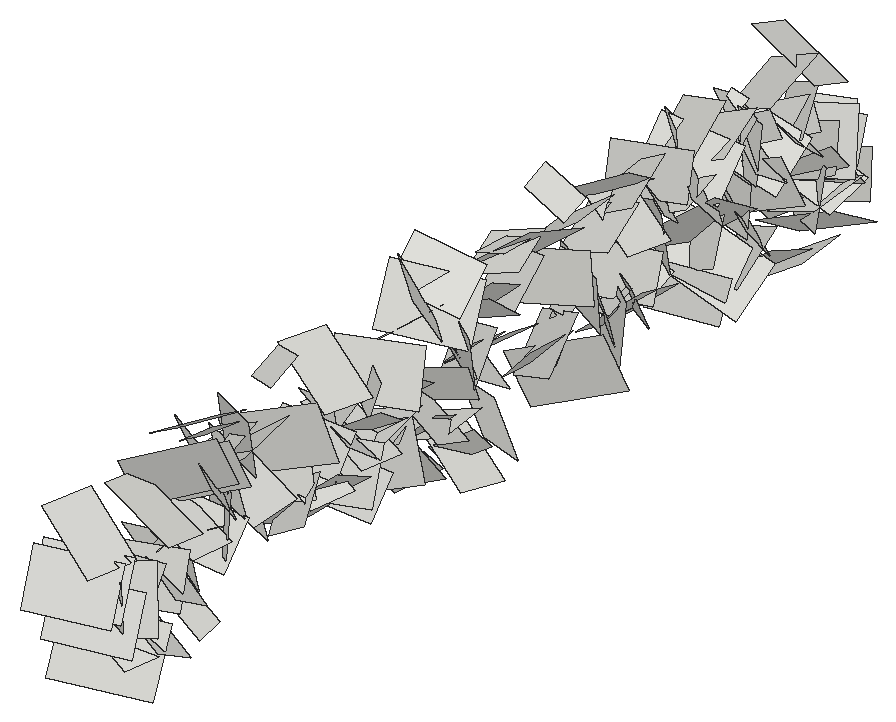
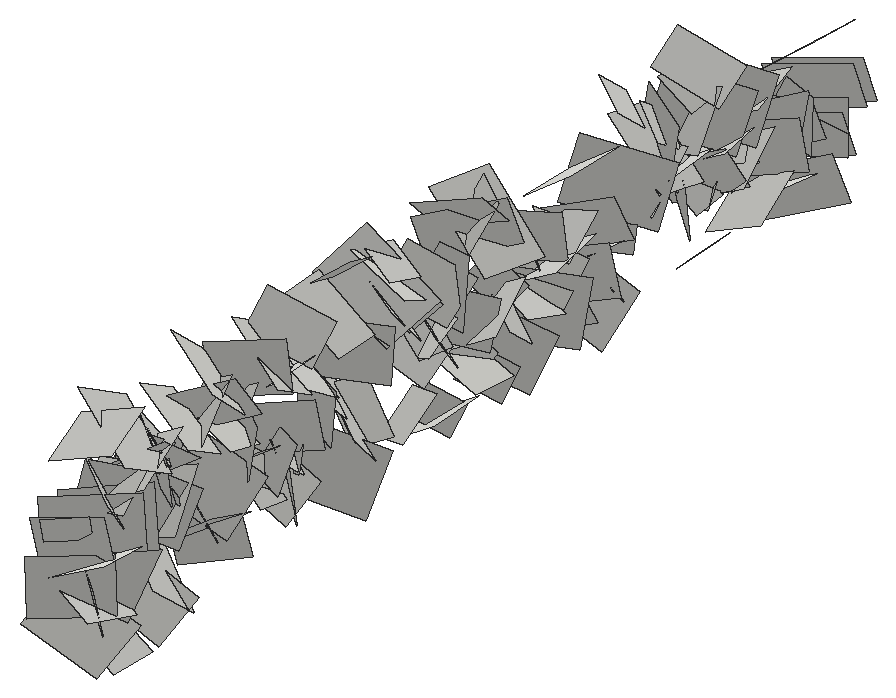
# SketchUp Ruby script. Lengths in inches.
U = 1.inch
M = Sketchup.active_model
def pt(a) = Geom::Point3d.new(a.map { |v| v * U })
def face(e, loops, mat)
  f = e.add_face(loops[0].map { |a| pt(a) })
  loops[1..].each { |l| e.add_face(l.map { |a| pt(a) }).erase! }
  f.material = f.back_material = mat if mat
  f
end
# faces: each face lists its corners as indices into pts; further lists are holes
def faces(e, pts, list, mat = nil) = list.each { |f| face(e, (f[0].is_a?(Array) ? f : [f]).map { |l| l.map { |i| pts[i] } }, mat) }
# xy, xz, yz: faces in a plane at the given z, y or x. An outline is a flat list of corners, or four numbers for a rectangle; further outlines are holes
def ring(l) = l.size == 4 ? [[l[0], l[1]], [l[2], l[1]], [l[2], l[3]], [l[0], l[3]]] : l.each_slice(2).to_a
def flat(e, list, mat, &to3) = list.each { |f| face(e, (f[0].is_a?(Array) ? f : [f]).map { |l| ring(l).map { |u, v| to3.(u, v) } }, mat) }
def xy(e, z, list, mat = nil) = flat(e, list, mat) { |x, y| [x, y, z] }
def xz(e, y, list, mat = nil) = flat(e, list, mat) { |x, z| [x, y, z] }
def yz(e, x, list, mat = nil) = flat(e, list, mat) { |y, z| [x, y, z] }
def lines(e, pts, list) = list.each { |a, b| e.add_line(pt(pts[a]), pt(pts[b])) }
# prism: a flat outline (further loops are holes) pulled along v
def prism(e, loops, v, mat = nil)
  f = face(e, loops, mat); d = Geom::Vector3d.new(v.map { |x| x * U })
  f.pushpull(f.normal.samedirection?(d) ? d.length : -d.length)
end
def box(e, o, s, mat = nil) = prism(e, [[o, [o[0] + s[0], o[1], o[2]], [o[0] + s[0], o[1] + s[1], o[2]], [o[0], o[1] + s[1], o[2]]]], [0, 0, s[2]], mat)
def at(x, y, z, deg = 0) = Geom::Transformation.translation(pt([x, y, z])) * Geom::Transformation.rotation(ORIGIN, Z_AXIS, deg.degrees)
def axes(o, x, y, z) = Geom::Transformation.new([*x, 0, *y, 0, *z, 0, *pt(o).to_a, 1])
def part(name) = M.definitions.add(name)
# library, detail: a bought-in or finely detailed component or shape, given as its bounding box
def library(name, o, s) = part(name).tap { |d| box(d.entities, o, s) }
def detail(e, o, s) = box(e.add_group.entities, o, s)
def put(e, d, t, mat = nil) = e.add_instance(d, t).tap { |i| i.material = mat if mat }
def group(e, t, mat = nil) = e.add_group.tap { |g| g.transformation = t; g.material = mat if mat }.entities
root = M.entities
c1 = part("Component\#6")
p = [[0.01,0,0],[0,3.24,4.54],[4.32,3.24,4.54],[4.33,0,0]]
faces(c1.entities,p,[[0,1,2,3]])
put(root,c1,axes([404.88,137.29,38.52],[0.00887,0.62519,-1.13199],[0.07674,-1.13046,-0.62381],[-1.3686,-0.05933,-0.04231]))
put(root,c1,axes([404.88,143.42,27.33],[-0.08667,-0.86973,1.01008],[0.23887,0.9884,0.86929],[-1.39256,0.22367,0.08625]))
put(root,c1,axes([404.88,132.16,25.41],[0.07094,-0.60211,-1.2376],[0.1162,-1.23279,0.6057],[-1.45423,-0.12788,-0.01197]))
put(root,c1,axes([404.88,172.47,36.95],[-0.1233,0.89549,0.4145],[-0.21728,0.38634,-0.89217],[-1.02316,-0.18996,0.13951]))
put(root,c1,axes([404.88,163.85,26.9],[-0.03329,1.04875,0.11229],[-0.24045,0.10299,-1.02538],[-1.09187,-0.05466,0.22238]))
put(root,c1,axes([404.88,195.34,33.06],[-0.01901,1.14103,-0.72029],[0.19621,-0.71146,-1.13165],[-1.41679,-0.11384,-0.14706]))
put(root,c1,axes([404.88,185.59,36.56],[-0.07365,1.00309,0.56692],[-0.00038,0.56794,-1.00493],[-1.22135,-0.06067,-0.03387]))
put(root,c1,axes([404.88,208.94,26.04],[0.1299,1.02121,-0.60997],[-0.25035,-0.5801,-1.01865],[-1.23578,0.22487,0.14225]))
put(root,c1,axes([404.88,141.2,30.22],[-0.14348,-0.5033,-0.91823],[-0.06175,-0.92081,0.51331],[-1.10823,0.11647,0.09028]))
put(root,c1,axes([404.88,196.35,35.86],[-0.06555,0.97369,0.5362],[-0.0688,0.53295,-0.97527],[-1.17625,-0.08544,0.02716]))
put(root,c1,axes([404.88,141.99,33.2],[-0.15631,-0.03731,1.01998],[-0.08418,1.02787,0.02612],[-1.07863,-0.07482,-0.14985]))
put(root,c1,axes([404.88,190.1,29],[-0.15352,-0.05709,1.12322],[0.06907,1.13017,0.06585],[-1.19015,0.07295,-0.14107]))
put(root,c1,axes([404.88,182.88,33.98],[-0.05541,0.90127,0.55592],[-0.17138,0.54328,-0.89597],[-1.1093,-0.12895,0.11065]))
put(root,c1,axes([404.88,146.73,29.36],[0.09029,-1.26195,0.03468],[-0.03892,0.03227,1.26436],[-1.33761,-0.08612,-0.03444]))
put(root,c1,axes([404.88,175.96,26.52],[-0.03553,0.82214,0.9074],[0.07429,0.90754,-0.81968],[-1.2958,0.02948,-0.07187]))
put(root,c1,axes([404.88,209.74,33.23],[-0.15201,0.07034,-1.21602],[0.20156,-1.20811,-0.09231],[-1.2753,-0.19933,0.13035]))
put(root,c1,axes([404.88,129.14,29.25],[0.07983,-0.47542,-1.06148],[-0.1788,-1.05692,0.46141],[-1.21984,0.1238,-0.1371]))
put(root,c1,axes([404.88,127.85,32.74],[0.07983,-0.47542,-1.06148],[-0.1788,-1.05692,0.46141],[-1.21984,0.1238,-0.1371]))
put(root,c1,axes([404.88,126.73,32.74],[0.07983,-0.47542,-1.06148],[-0.1788,-1.05692,0.46141],[-1.21984,0.1238,-0.1371]))
put(root,c1,axes([404.88,156.79,29.67],[-0.01777,-0.29003,-1.18393],[0.05362,-1.18318,0.28913],[-1.29096,-0.04516,0.0283]))
put(root,c1,axes([404.88,155.57,33.875],[-0.13701,-1.11756,0.11199],[0.07264,0.10468,1.12363],[-1.18833,0.13525,0.05577]))
put(root,c1,axes([404.88,151.45,29.33],[-0.11063,1.17252,-0.59491],[0.28501,-0.56514,-1.16101],[-1.36425,-0.21315,-0.19431]))
put(root,c1,axes([404.88,134.27,30.6],[-0.0256,-0.22889,-1.14247],[-0.00761,-1.14266,0.22909],[-1.23506,0.01178,0.02227]))
put(root,c1,axes([404.88,182.25,27.43],[0.1955,0.46825,-1.21407],[-0.10064,-1.21809,-0.48422],[-1.37564,0.15566,-0.13711]))
put(root,c1,axes([404.88,204.59,30.02],[0.04301,-1.09683,0.72238],[0.12053,0.72294,1.0913],[-1.38692,0.02882,0.11724]))
put(root,c1,axes([404.88,149.09,36.34],[0.1737,0.35213,-1.24285],[-0.08,-1.24806,-0.36356],[-1.36694,0.11779,-0.13666]))
put(root,c1,axes([404.88,180.75,35.09],[0.01445,0.08276,-1.11066],[-0.1396,-1.10283,-0.0838],[-1.17228,0.13235,-0.00371]))
put(root,c1,axes([404.88,201.85,37.73],[0.10519,1.13817,0.58904],[0.00109,0.59073,-1.14161],[-1.35845,0.08861,0.0447]))
put(root,c1,axes([404.88,198.78,35.93],[-0.06513,-0.64723,-0.92238],[-0.00055,-0.92374,0.64822],[-1.19442,0.03572,0.05]))
put(root,c1,axes([404.88,181.98,27.65],[-0.03848,-0.07343,1.06513],[-0.13392,1.05855,0.06867],[-1.12376,-0.12364,-0.04466]))
put(root,c1,axes([404.88,200.11,31.93],[-0.08158,0.26048,1.04137],[-0.05734,1.04178,-0.26458],[-1.13642,-0.07126,-0.06141]))
put(root,c1,axes([400.91,188.74,27.6],[-0.13014,-0.45431,-0.37588],[-0.00674,-0.3829,0.46487],[0.62498,-0.09873,-0.07326]))
put(root,c1,axes([404.88,153.58,31.99],[-0.17505,-0.32324,-0.90395],[-0.10086,-0.9072,0.34179],[-1.0126,0.14624,0.12223]))
put(root,c1,axes([400.91,136.62,23.89],[-0.08859,0.63974,0.04756],[-0.12242,0.03217,-0.63572],[0.66888,0.09062,-0.11005]))
put(root,c1,axes([404.88,213.06,27.02],[0.109,-1.16412,-0.17966],[-0.1638,-0.19212,1.15639],[-1.23778,-0.07709,-0.16885]))
put(root,c1,axes([404.88,137.65,40.3125],[-0.15365,0.92766,-0.3555],[-0.07441,-0.36793,-0.93147],[-1.05042,-0.10963,0.11798]))
put(root,c1,axes([404.88,201.95,25.76],[-0.02109,1.10253,-0.4508],[0.04504,-0.44992,-1.10225],[-1.2618,-0.03449,-0.03181]))
put(root,c1,axes([404.88,140.69,35.43],[-0.02714,1.22478,0.26938],[0.1382,0.27058,-1.21783],[-1.3221,0.00314,-0.13283]))
put(root,c1,axes([404.88,128.2,32.33],[-0.15852,-1.12421,0.05612],[0.12401,0.04078,1.12872],[-1.18668,0.15444,0.11046]))
put(root,c1,axes([404.88,138.43,27.8],[-0.10648,0.28124,1.16655],[0.16097,1.1642,-0.2676],[-1.26174,0.12479,-0.13259]))
put(root,c1,axes([404.88,157.84,26.69],[-0.16666,-0.37984,-0.88441],[-0.10341,-0.88523,0.39754],[-1.01503,0.15255,0.10471]))
put(root,c1,axes([404.88,213.59,29.33],[-0.10669,0.07311,-1.12569],[0.06812,-1.12796,-0.079],[-1.19381,-0.0709,0.09609]))
put(root,c1,axes([404.88,160.05,30.35],[0.12426,0.20575,-1.35522],[0.11745,-1.35714,-0.19646],[-1.44825,-0.0924,-0.13221]))
put(root,c1,axes([404.88,158.93,27.77],[0.0679,-1.16178,0.21088],[-0.08573,0.20637,1.16154],[-1.24867,-0.07734,-0.06828]))
put(root,c1,axes([404.88,192.86,38.11],[-0.10772,-0.0541,-1.0459],[-0.04447,-1.04976,0.05837],[-1.10925,0.04734,0.09923]))
put(root,c1,axes([400.91,172.58,29],[-0.14706,-0.68518,0.03236],[-0.10474,0.05263,0.69082],[0.71951,-0.13238,0.10718]))
put(root,c1,axes([404.88,208.81,31.45],[0.04602,0.84125,-1.04893],[0.18208,-1.04435,-0.83047],[-1.4136,-0.10713,-0.14111]))
put(root,c1,axes([404.88,168.84,39.14],[-0.0295,-0.69575,-0.73723],[-0.22295,-0.71749,0.68506],[-1.05113,0.17171,-0.12461]))
put(root,c1,axes([404.88,187.65,25.55],[-0.14301,-0.32766,0.90945],[-0.11586,0.91755,0.31436],[-1.01811,-0.05839,-0.16352]))
put(root,c1,axes([404.88,167.41,29.34],[0.20833,-0.42173,1.22713],[-0.0869,1.23461,0.43743],[-1.37269,-0.14217,0.15855]))
put(root,c1,axes([404.88,163.625,35.04],[-0.27654,-0.44632,0.88094],[0.09901,0.89592,0.48157],[-1.04211,0.20356,-0.18801]))
put(root,c1,axes([404.88,202.23,24.6],[0.19755,-1.2824,-0.48224],[0.04087,-0.48158,1.29554],[-1.4517,-0.18807,-0.02915]))
put(root,c1,axes([404.88,153.43,27.14],[-0.15407,-0.97446,-0.01303],[-0.08051,-0.00181,0.98239],[-1.02988,0.14592,-0.07485]))
put(root,c1,axes([404.88,147.58,26.68],[-0.22766,0.71104,0.67114],[0.02672,0.69094,-0.72395],[-1.03608,-0.13842,-0.16614]))
put(root,c1,axes([400.91,203.75,35.72],[-0.12855,-0.35471,-0.52952],[-0.05195,-0.53223,0.36775],[0.67359,-0.10874,-0.07269]))
put(root,c1,axes([404.88,192.77,37.47],[0.01566,0.85002,0.74451],[-0.07038,0.74394,-0.84805],[-1.19569,-0.03266,0.05967]))
put(root,c1,axes([400.91,163.13,28.77],[-0.13219,-0.55975,0.33448],[-0.05965,0.34851,0.56225],[0.68862,-0.07726,0.11291]))
put(root,c1,axes([404.88,197.22,25.56],[-0.17769,-0.12121,-0.94504],[-0.07151,-0.95564,0.13453],[-1.00742,0.08922,0.15714]))
put(root,c1,axes([404.88,130.48,31.34],[0.20009,-0.24055,-1.32848],[0.01815,-1.34087,0.24522],[-1.43098,-0.05064,-0.18264]))
put(root,c1,axes([404.88,210.75,36.02],[0.14272,-1.0645,0.43866],[-0.22696,0.41079,1.0626],[-1.19913,-0.20445,-0.14891]))
put(root,c1,axes([404.88,205.38,23.16],[-0.04798,1.09948,0.05597],[-0.01409,0.05547,-1.10036],[-1.16688,-0.04588,0.01099]))
put(root,c1,axes([404.88,139.23,29.07],[0.06497,-1.13195,0.1646],[-0.10003,0.15928,1.13044],[-1.20835,-0.07404,-0.08473]))
put(root,c1,axes([404.88,161.68,35.57],[0.09547,-0.29138,-1.10436],[-0.14499,-1.10257,0.27976],[-1.20197,0.10985,-0.12146]))
put(root,c1,axes([400.91,191.07,24.72],[-0.08022,-0.60182,-0.03468],[-0.03515,-0.03074,0.60586],[0.63802,-0.07736,0.02902]))
put(root,c1,axes([404.88,171.44,27.64],[-0.05126,-0.8571,0.56567],[-0.11133,0.56746,0.85083],[-1.08285,-0.01777,-0.11425]))
put(root,c1,axes([404.88,173.84,39.64],[0.13369,1.27699,-0.41872],[0.11509,-0.42887,-1.27523],[-1.41986,0.08547,-0.14279]))
put(root,c1,axes([400.91,202.49,32.61],[-0.11645,-0.17214,0.59947],[-0.01233,0.60916,0.17278],[0.661,-0.01896,0.10883]))
put(root,c1,axes([404.88,134.42,21.5625],[0.1234,-1.02964,0.56694],[-0.11588,0.55776,1.03542],[-1.24053,-0.15452,-0.04032]))
put(root,c1,axes([404.88,156.69,29.48],[0.02364,1.01192,0.31394],[-0.16386,0.31376,-1.00035],[-1.11105,-0.02474,0.15421]))
put(root,c1,axes([404.88,206.95,24.98],[-0.09414,0.39654,1.07266],[0.12922,1.07305,-0.38659],[-1.20532,0.08407,-0.12522]))
put(root,c1,axes([400.91,173.74,31.89],[-0.15856,-0.67469,0.29232],[-0.1064,0.31425,0.67394],[0.77211,-0.09525,0.1529]))
put(root,c1,axes([400.91,147.9,27.03],[-0.12769,0.03013,0.63893],[-0.01482,0.64988,-0.03329],[0.67785,0.01989,0.11963]))
put(root,c1,axes([400.91,181.39,28.46],[-0.11732,-0.15238,-0.58962],[0.01785,-0.59981,0.15186],[0.64528,-0.01111,-0.1114]))
put(root,c1,axes([404.88,131.47,30.67],[-0.19347,-0.24403,-0.96391],[0.05093,-0.98104,0.23927],[-1.05275,-0.00261,0.18872]))
put(root,c1,axes([404.88,139.67,30.68],[0.09112,-0.77438,0.96294],[0.03313,0.96632,0.77431],[-1.3094,-0.02944,0.0866]))
put(root,c1,axes([404.88,167.53,29.6],[-0.04916,0.6172,0.8297],[-0.08211,0.82613,-0.61887],[-1.09305,-0.08981,0.00917]))
put(root,c1,axes([400.91,137.74,29.49],[-0.05063,0.39266,-0.56355],[-0.15447,-0.55784,-0.37633],[0.71149,-0.09317,-0.12181]))
put(root,c1,axes([404.88,195.04,27.27],[-0.2131,0.57774,0.71728],[-0.02179,0.73117,-0.59469],[-0.97604,-0.14247,-0.14333]))
put(root,c1,axes([404.88,211.99,33.59],[0.13241,-0.25962,-1.28668],[0.09489,-1.2878,0.26854],[-1.38813,-0.1128,-0.10438]))
put(root,c1,axes([404.88,170.89,20.28],[-0.12274,-1.02279,0.17958],[0.0333,0.17716,1.02926],[-1.10024,0.11946,0.01112]))
put(root,c1,axes([404.88,206.8125,26.89],[0.15204,1.11982,0.24611],[-0.19339,0.26716,-1.10927],[-1.19986,0.09884,0.20998]))
put(root,c1,axes([400.91,144.97,35.07],[-0.07722,-0.5315,-0.34657],[-0.05738,-0.34237,0.53643],[0.67013,-0.09056,0.006]))
put(root,c1,axes([404.88,206.55,33.15],[-0.00164,-0.95203,-0.71322],[0.09471,-0.7113,0.94927],[-1.25737,-0.05234,0.07244]))
put(root,c1,axes([400.91,140.39,26.94],[-0.03872,-0.62994,0.14227],[-0.11345,0.14643,0.62088],[0.67508,-0.01152,0.1125]))
put(root,c1,axes([404.88,189.26,31.29],[-0.07003,-0.18149,-1.00879],[-0.05402,-1.00905,0.18487],[-1.08514,0.06195,0.0559]))
put(root,c1,axes([404.88,201.66,25.46],[0.21728,-0.88431,0.94199],[-0.03627,0.94972,0.89901],[-1.36907,-0.16551,0.12568]))
put(root,c1,axes([404.88,131.52,23.18],[-0.15485,-0.9106,-0.00305],[-0.11373,0.01414,0.91588],[-0.95852,0.14543,-0.10818]))
put(root,c1,axes([404.88,169.04,36.23],[0.04162,0.78981,-0.64322],[-0.24351,-0.62024,-0.77563],[-1.05189,0.17484,0.15411]))
put(root,c1,axes([400.91,163.1,21.29],[-0.03251,-0.459,0.52355],[-0.17075,0.51451,0.44164],[0.71801,0.10157,0.12873]))
put(root,c1,axes([404.88,184.16,23.6],[-0.00632,0.19994,1.20323],[0.15077,1.19515,-0.1979],[-1.28409,0.13934,-0.02916]))
put(root,c1,axes([404.88,158.58,28.72],[-0.17742,0.80309,0.64454],[0.10421,0.66248,-0.79991],[-1.08655,-0.0676,-0.18196]))
put(root,c1,axes([404.88,168.75,37.98],[0.06882,-0.53698,-1.12739],[0.1022,-1.12338,0.54063],[-1.31971,-0.115,-0.01692]))
put(root,c1,axes([400.91,210.56,30.82],[-0.08988,0.23539,0.56706],[0.00516,0.57268,-0.23699],[0.65079,0.02797,0.0802]))
put(root,c1,axes([404.88,156.02,28.65],[0.0619,-0.85924,0.62732],[-0.17366,0.61351,0.85557],[-1.11425,-0.14335,-0.09849]))
put(root,c1,axes([400.91,160.09,33.87],[-0.13785,-0.16653,-0.67513],[-0.04892,-0.68326,0.17743],[0.73546,-0.07666,-0.11474]))
put(root,c1,axes([400.91,206,31.6],[-0.1462,-0.08624,0.716],[-0.07336,0.72719,0.07426],[0.76092,0.05354,0.14472]))
put(root,c1,axes([400.91,183.51,30.36],[-0.10644,-0.42009,-0.4575],[0.01901,-0.46521,0.42323],[0.65811,-0.0545,-0.08622]))
put(root,c1,axes([400.91,191.45,35.51],[-0.13227,0.51495,-0.41011],[-0.00116,-0.41758,-0.52399],[0.6978,0.09692,-0.07861]))
put(root,c1,axes([404.88,156.45,32.24],[-0.14884,0.843,-0.57449],[0.06248,-0.57223,-0.85409],[-1.07954,-0.14935,0.02978]))
put(root,c1,axes([404.88,202.95,33.21],[0.17447,0.42234,-1.07867],[-0.17991,-1.06896,-0.44444],[-1.21466,0.21899,-0.08911]))
put(root,c1,axes([404.88,126.5625,26.98],[0.04661,-0.13743,1.04442],[-0.16266,1.03335,0.14244],[-1.10472,-0.15795,0.02309]))
put(root,c1,axes([400.91,136.41,29.65],[-0.07813,-0.63244,-0.26103],[-0.10098,-0.25049,0.63382],[0.71818,-0.10402,0.06072]))
put(root,c1,axes([400.91,157.4,31.875],[-0.05779,-0.51798,-0.36432],[-0.0587,-0.36037,0.52065],[0.6687,-0.0764,0.01422]))
put(root,c1,axes([404.88,179.35,38.14],[-0.07028,1.07405,0.02302],[0.04111,0.02544,-1.07534],[-1.13802,-0.06541,-0.04027]))
put(root,c1,axes([404.88,199.05,27.98],[-0.08019,0.19915,0.92966],[-0.13728,0.92174,-0.20799],[-0.9984,-0.14274,-0.04607]))
put(root,c1,axes([404.88,207.91,30.98],[0.03881,-0.77727,0.6188],[-0.26695,0.59174,0.75817],[-1.01873,-0.18467,-0.1751]))
put(root,c1,axes([404.88,166.67,25.47],[0.29316,-1.18227,0.54308],[-0.10516,0.53443,1.21398],[-1.37509,-0.29293,0.02294]))
put(root,c1,axes([404.88,171.47,32.36],[-0.16942,0.96147,-0.31887],[0.08969,-0.30901,-0.97416],[-1.06999,-0.17814,-0.03117]))
put(root,c1,axes([400.91,149.56,39.6],[-0.17317,-0.50739,-0.45031],[0.03865,-0.46908,0.51531],[0.71806,-0.09712,-0.13634]))
put(root,c1,axes([400.91,169.1,21.1],[-0.05323,-0.42134,0.48328],[-0.06346,0.48572,0.41725],[0.67666,0.01241,0.07715]))
put(root,c1,axes([404.88,135.84,31.22],[0.16391,-1.12855,0.28901],[-0.13375,0.27361,1.13591],[-1.2276,-0.1805,-0.08517]))
put(root,c1,axes([404.88,186.92,28.87],[-0.11772,1.08189,-0.3436],[0.18933,-0.32428,-1.0788],[-1.18826,-0.15885,-0.13785]))
put(root,c1,axes([404.88,166.55,31.56],[-0.0814,0.41102,-0.8284],[-0.17089,-0.82447,-0.39413],[-0.96524,0.11131,0.13964]))
put(root,c1,axes([404.88,185.29,39.56],[-0.11827,0.82487,-0.51088],[-0.03346,-0.51706,-0.82795],[-1.02793,-0.07808,0.08573]))
put(root,c1,axes([400.91,165.91,24.52],[0.03596,-0.58924,0.24858],[-0.15481,0.23521,0.57749],[0.65999,0.08727,0.12191]))
put(root,c1,axes([404.88,172.46,21.25],[-0.14489,-0.73421,0.72244],[0.08794,0.71856,0.74596],[-1.0883,0.15581,-0.0359]))
put(root,c1,axes([404.88,136.25,25.03],[0.1909,-1.05424,0.65515],[-0.04228,0.65676,1.06778],[-1.31502,-0.17416,0.06077]))
put(root,c1,axes([404.88,205.46,33.43],[-0.14097,0.63084,0.7943],[0.06243,0.80455,-0.62912],[-1.07339,-0.03606,-0.14091]))
put(root,c1,axes([404.88,197.83,24.35],[0.09568,0.96283,0.81475],[0.1112,0.80827,-0.9668],[-1.33234,0.1366,-0.02218]))
put(root,c1,axes([404.88,138.81,37.71],[0.08326,0.50336,-1.07522],[0.02589,-1.07803,-0.50289],[-1.25818,0.01113,-0.0815]))
put(root,c1,axes([400.91,180.42,25.12],[-0.17902,-0.88337,-0.09354],[-0.21931,-0.05348,0.8786],[0.91571,-0.1855,0.19214]))
put(root,c1,axes([400.91,176.07,37.03],[-0.15674,-0.62528,-0.09698],[0.10666,-0.12156,0.63036],[0.66219,-0.12843,-0.12449]))
put(root,c1,axes([400.91,188.83,29.07],[-0.04972,0.59189,0.16701],[-0.02122,0.16593,-0.59371],[0.65156,0.05057,-0.00659]))
put(root,c1,axes([404.88,212.99,32.26],[-0.05541,-0.21084,-0.92918],[-0.15034,-0.91849,0.21639],[-0.99872,0.14996,0.01898]))
put(root,c1,axes([400.91,141.05,35.76],[-0.06877,-0.60814,0.14272],[-0.00885,0.14432,0.61116],[0.66208,-0.06124,0.02299]))
put(root,c1,axes([404.88,171.95,33.74],[0.07102,0.70639,0.8167],[-0.11892,0.8184,-0.69866],[-1.13841,-0.04142,0.12393]))
put(root,c1,axes([404.88,159.57,38.3125],[0.19748,1.37219,0.09956],[0.15298,0.08042,-1.37849],[-1.4503,0.19533,-0.13185]))
put(root,c1,axes([404.88,160.7,27.63],[0.09928,0.64406,-0.88513],[-0.13228,-0.87629,-0.65083],[-1.15276,0.15602,-0.00154]))
put(root,c1,axes([404.88,190.19,31.82],[-0.07854,-1.04848,0.11995],[0.05802,0.11627,1.05008],[-1.11713,0.07975,0.0461]))
put(root,c1,axes([400.91,178.13,40.15],[-0.04908,0.64392,0.19174],[-0.08573,0.18545,-0.64234],[0.70699,0.06719,-0.06458]))
put(root,c1,axes([400.91,186.02,29.02],[-0.12909,0.32312,-0.64935],[-0.06195,-0.66067,-0.31779],[0.76632,0.00102,-0.13508]))
put(root,c1,axes([404.88,191.97,33.56],[-0.08688,0.89449,0.25558],[-0.12211,0.24484,-0.89383],[-0.97851,-0.10998,0.08885]))
put(root,c1,axes([404.88,196.22,30.25],[0.08073,-0.93811,0.99109],[0.27356,0.98462,0.91216],[-1.42044,0.13631,0.232]))
